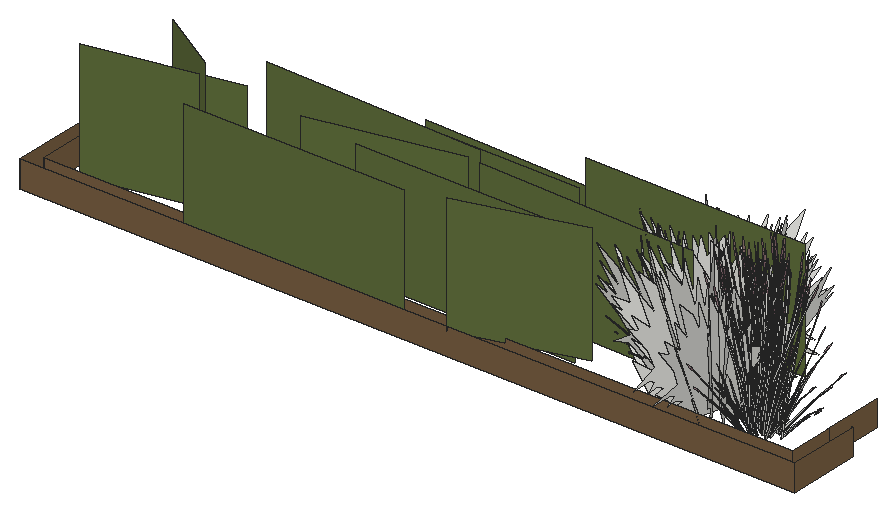
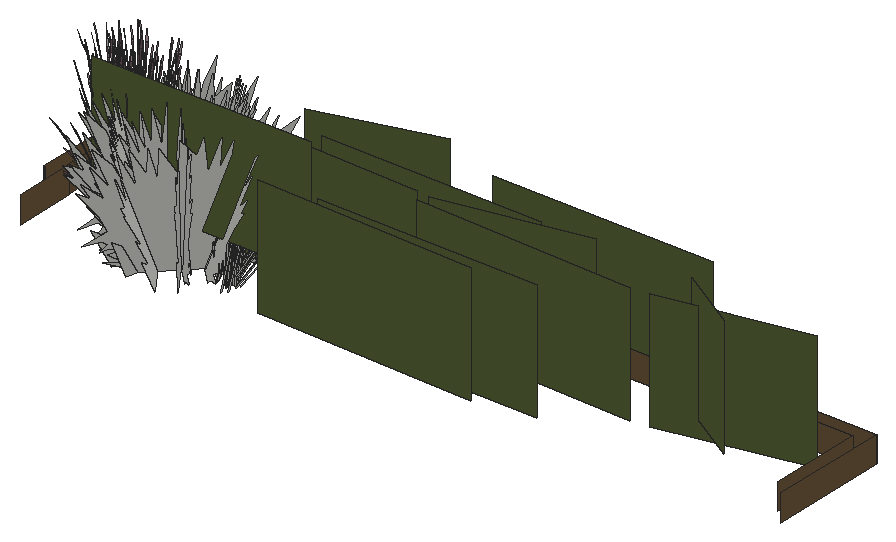
# SketchUp Ruby script. Lengths in inches.
U = 1.inch
M = Sketchup.active_model
def pt(a) = Geom::Point3d.new(a.map { |v| v * U })
def face(e, loops, mat)
  f = e.add_face(loops[0].map { |a| pt(a) })
  loops[1..].each { |l| e.add_face(l.map { |a| pt(a) }).erase! }
  f.material = f.back_material = mat if mat
  f
end
# faces: each face lists its corners as indices into pts; further lists are holes
def faces(e, pts, list, mat = nil) = list.each { |f| face(e, (f[0].is_a?(Array) ? f : [f]).map { |l| l.map { |i| pts[i] } }, mat) }
# xy, xz, yz: faces in a plane at the given z, y or x. An outline is a flat list of corners, or four numbers for a rectangle; further outlines are holes
def ring(l) = l.size == 4 ? [[l[0], l[1]], [l[2], l[1]], [l[2], l[3]], [l[0], l[3]]] : l.each_slice(2).to_a
def flat(e, list, mat, &to3) = list.each { |f| face(e, (f[0].is_a?(Array) ? f : [f]).map { |l| ring(l).map { |u, v| to3.(u, v) } }, mat) }
def xy(e, z, list, mat = nil) = flat(e, list, mat) { |x, y| [x, y, z] }
def xz(e, y, list, mat = nil) = flat(e, list, mat) { |x, z| [x, y, z] }
def yz(e, x, list, mat = nil) = flat(e, list, mat) { |y, z| [x, y, z] }
def lines(e, pts, list) = list.each { |a, b| e.add_line(pt(pts[a]), pt(pts[b])) }
# prism: a flat outline (further loops are holes) pulled along v
def prism(e, loops, v, mat = nil)
  f = face(e, loops, mat); d = Geom::Vector3d.new(v.map { |x| x * U })
  f.pushpull(f.normal.samedirection?(d) ? d.length : -d.length)
end
def box(e, o, s, mat = nil) = prism(e, [[o, [o[0] + s[0], o[1], o[2]], [o[0] + s[0], o[1] + s[1], o[2]], [o[0], o[1] + s[1], o[2]]]], [0, 0, s[2]], mat)
def at(x, y, z, deg = 0) = Geom::Transformation.translation(pt([x, y, z])) * Geom::Transformation.rotation(ORIGIN, Z_AXIS, deg.degrees)
def axes(o, x, y, z) = Geom::Transformation.new([*x, 0, *y, 0, *z, 0, *pt(o).to_a, 1])
def part(name) = M.definitions.add(name)
# library, detail: a bought-in or finely detailed component or shape, given as its bounding box
def library(name, o, s) = part(name).tap { |d| box(d.entities, o, s) }
def detail(e, o, s) = box(e.add_group.entities, o, s)
def put(e, d, t, mat = nil) = e.add_instance(d, t).tap { |i| i.material = mat if mat }
def group(e, t, mat = nil) = e.add_group.tap { |g| g.transformation = t; g.material = mat if mat }.entities
root = M.entities
M.materials.add("Grass2").color = [97, 112, 61]
M.materials.add("LightPink_Translucent").color = [144, 107, 117]
M.materials["LightPink_Translucent"].alpha = 0.75
M.materials.add("Soil_03_1K").color = [122, 96, 67]
c1 = part("blade")
p = [[2.15,0.21,22],[0,0.17,0],[0.09,0.45,0],[2.18,0.31,22],[2.29,0.31,22],[0.38,0.45,0],
  [2.48,0.24,33],[2.49,0.24,33],[2.48,0.22,33]]
faces(c1.entities,p,[[0,1,2,3],[4,5,2,3],[6,3,4,7],[8,0,3,6]])
c2 = part("seeds")
p = [[0.3,-0.1,1.38],[-0.01,-0.03,1.59],[-0.01,-0.03,0.03],[0.14,-0.07,-0.07],[0.29,-0.03,3],[0.15,0.01,3.11]]
faces(c2.entities,p,[[0,1,2,3],[1,0,4,5]],"LightPink_Translucent")
c3 = part("blade with seeds")
put(c3.entities,c1,at(0,0,0))
put(c3.entities,c2,axes([2.4,0.25,30.99],[1.5799,-0.05474,1.17369],[-0.12525,1.92788,0.29478],[-0.07173,-0.02425,1.56792]))
c4 = part("Group\#22")
xz(c4.entities,0,[[0,0,62.37,62.37]],"Grass2")
c5 = part("Grass")
put(c5.entities,c4,at(102.75,113.61,7.86,-130.817))
put(c5.entities,c4,at(63.84,171.21,0.17))
put(c5.entities,c4,at(131.2,149.2,20.75))
put(c5.entities,c4,at(113.26,0,11.94,57.296))
put(c5.entities,c4,at(36.98,10.45,5.02))
put(c5.entities,c4,at(77.99,64.03,5.18))
put(c5.entities,c4,at(168.32,102.22,8.04,171.887))
put(c5.entities,c4,at(142.1,179.07,0,171.887))
put(c5.entities,c4,at(103.38,132.8,9.02,171.887))
put(c5.entities,c4,at(40.77,108.39,1.9,-130.817))
put(c5.entities,c4,at(14.86,142.73,10.93,-73.521))
c6 = part("blade with seeds\#1")
put(c6.entities,c1,at(0,0,0))
c7 = part("Component\#6")
xz(c7.entities,0,[[-7.84,0,-9.38,1.27,-13.33,2.74,-9.72,2.74,-12.46,4.76,-10.42,5.61,-11.09,5.91,-12.29,6.43,-14.04,5.51,-12.66,7.47,-13.79,8.27,-17.41,7.2,-12.68,10.6,-14.36,14.66,-18.8125,20.79,-16.1,19.31,-17.89,23.09,-13.72,19.25,-16.46,27.33,-12.55,21.85,-16.26,31.69,-12.42,27.71,-10.09,22.64,-11.66,30.3,-7.6,21.37,-9.33,31.16,-5.98,24.77,-5.98,31.16,-3.85,22.89,-3.85,31.16,-0.14,24.32,-0.14,32.95,3.15,28.93,4.22,33.24,5.28,24.41,7.5,33.04,7.5,25.47,9.76,32.21,9.01,24.9375,12.04,31.72,9.8,23.08,13.59,31.68,12.3,26.01,15.16,30.22,11.37,20.82,13.73,24.07,13.73,18.79,18.81,26.9375,17.03,20.08,20.56,21.75,18.25,18.3,20.56,20.08,12.54,9.27,16.8,12.66,11.125,4.45,16.74,8.03,13.47,0]])
c8 = part("Component\#7")
xz(c8.entities,0,[[-7.84,0,-9.38,1.27,-13.33,2.74,-9.72,2.74,-12.46,4.76,-10.42,5.61,-11.09,5.91,-12.29,6.43,-14.04,5.51,-12.66,7.47,-13.79,8.27,-17.41,7.2,-12.68,10.6,-14.36,14.66,-18.8125,20.79,-16.1,19.31,-17.89,23.09,-13.72,19.25,-16.46,27.33,-12.55,21.85,-16.26,31.69,-12.42,27.71,-10.09,22.64,-11.66,30.3,-7.6,21.37,-9.33,31.16,-5.98,24.77,-5.98,31.16,-3.85,22.89,-3.85,31.16,-0.14,24.32,-0.14,32.95,3.15,28.93,4.22,33.24,5.28,24.41,7.5,33.04,7.5,25.47,9.76,32.21,9.01,24.9375,12.04,31.72,9.8,23.08,13.59,31.68,12.3,26.01,15.16,30.22,11.37,20.82,13.73,24.07,13.73,18.79,18.81,26.9375,17.03,20.08,20.56,21.75,18.25,18.3,20.56,20.08,12.54,9.27,16.8,12.66,11.125,4.45,16.74,8.03,13.47,0]])
put(c8.entities,c7,axes([0,-4.21,0],[1,0,0],[0,0.96593,0.25882],[0,-0.25882,0.96593]))
c9 = part("Ornamental grass clump")
put(c9.entities,c8,axes([-3.36,-0.02,0],[1.6215,0,0],[0,1.6215,0],[0,0,1.6215]))
put(c9.entities,c8,axes([-0.07,-1.84,0],[-0.93005,1.32826,0],[-1.32826,-0.93005,0],[0,0,1.6215]))
put(c9.entities,c8,axes([1.16,1.19,0],[-1.14657,-1.14657,0],[1.14657,-1.14657,0],[0,0,1.6215]))
put(c9.entities,c8,axes([-0.28,-3,0],[0.41968,1.56625,0],[-1.56625,0.41968,0],[0,0,1.6215]))
put(c9.entities,c8,axes([-2.07,1.56,0],[1.14657,-1.14657,0],[1.14657,1.14657,0],[0,0,1.6215]))
xz(root,49.75,[[307.48,0,600.39,10]],"Soil_03_1K")
xz(root,54.75,[[312.48,0,595.39,10]],"Soil_03_1K")
xz(root,71.87,[[595,0,595.39,10]])
xz(root,76.87,[[600,0,600.39,10]])
yz(root,307.48,[[49.75,0,94.87,10]],"Soil_03_1K")
yz(root,312.48,[[54.75,0,89.87,10]],"Soil_03_1K")
yz(root,595,[[71.87,0,94.87,10]],"Soil_03_1K")
yz(root,595.39,[[54.75,0,71.87,10]],"Soil_03_1K")
yz(root,600.39,[[49.75,0,76.87,10]],"Soil_03_1K")
put(root,c3,axes([572.64,67.23,1.78],[-0.34835,0.20963,1.43002],[-1.04325,-0.36691,-0.30754],[0.19338,-0.4563,0.61141]))
put(root,c3,axes([567.24,66.83,1.78],[-0.07421,0.33879,1.43002],[-1.08488,0.28361,-0.30754],[-0.25359,-0.4379,0.61141]))
put(root,c3,axes([570.04,66.09,0.6875],[-0.20555,0.03731,1.76342],[-1.13672,-0.42002,-0.26939],[0.01907,-0.35034,0.30037]))
put(root,c3,axes([571.35,65.56,1.96],[0.15721,0.60392,1.1486],[-0.87211,-0.33448,0.84392],[0.09385,-0.30923,0.25299]))
put(root,c3,axes([566.87,66.29,1.96],[0.63926,0.36046,1.1486],[-0.93099,0.21668,0.84392],[-0.1992,-0.27702,0.25299]))
put(root,c3,axes([566.36,67.37,0.6875],[-0.11871,0.13643,1.76342],[-1.19964,0.29415,-0.26939],[-0.2898,-0.26759,0.30037]))
put(root,c3,axes([568.34,71.12,1.29],[-0.50328,-1.06202,-0.69835],[1.44974,-0.38248,-0.18329],[-0.05563,-0.35963,1.54149]))
put(root,c3,axes([575.07,67.875,0.6875],[-0.18342,-0.08159,1.76342],[-0.47115,-0.9115,-0.26939],[0.31784,-0.24736,0.30037]))
put(root,c3,axes([568.14,68.07,1.57],[-0.7662,-1.03778,0],[1.28187,-0.57875,-0.51607],[0.29196,-0.13181,1.63711]))
put(root,c3,axes([569.83,66.82,1.32],[-0.84686,0.59414,-0.03893],[-0.77596,-0.65071,-0.17649],[-0.05463,-0.18438,0.58215]))
put(root,c3,axes([565.375,70.97,1.21],[0,-1.03566,-0.49651],[1.37109,0,0],[0,-0.23588,1.57504]))
put(root,c3,axes([569.1875,67.91,1.21],[1.14694,-0.51783,-0.49651],[0.68554,0.92854,0],[0.26122,-0.11794,1.57504]))
put(root,c3,axes([575.99,69.7,1.78],[-0.4378,-0.03068,1.43002],[-0.44851,-0.8229,-0.30754],[0.53783,-0.23279,0.61141]))
put(root,c3,axes([570.55,70.03,1.25],[0.82544,-0.77843,-0.62353],[1.0254,0.70586,-0.16365],[0.33076,-0.19418,1.37633]))
put(root,c3,axes([576.5,68.18,1.96],[-0.40819,0.5272,1.1486],[-0.35086,-0.70831,0.84392],[0.33713,-0.17749,0.25299]))
put(root,c3,axes([569.11,71.4,1.4],[0.59459,-0.93321,-0.44739],[1.23546,0.44912,0.21531],[0,-0.21512,1.43643]))
put(root,c3,axes([569.65,70.93,1.86],[-0.1428,-1.18174,-0.29095],[1.48733,-0.07145,-0.50002],[0.26191,-0.15741,1.59708]))
put(root,c3,axes([565.96,71,1.22],[0.85545,-0.64616,-0.30978],[0.85545,0.64616,0.30978],[0,-0.20813,1.38974]))
put(root,c3,axes([565.62,67.9,1.32],[-0.35352,0.84566,-0.03893],[-1.08806,-0.26014,-0.17649],[-0.1652,-0.13832,0.58215]))
put(root,c3,axes([568.96,72.17,1.86],[-1.38012,-0.49416,-0.29095],[0.66454,-1.04299,-0.50002],[-0.04337,-0.25608,1.59708]))
put(root,c3,axes([565.03,71.76,1.57],[-1.53239,0,0],[0,-1.1575,-0.51607],[0,-0.26363,1.63711]))
put(root,c3,axes([565.29,69.69,1.78],[0.23927,0.28834,1.43002],[-0.55135,0.78376,-0.30754],[-0.56612,-0.18733,0.61141]))
put(root,c3,axes([569.45,68.32,1.22],[1.14332,0.25625,-0.30978],[-0.28787,0.90242,0.30978],[0.23049,-0.10406,1.38974]))
put(root,c3,axes([566.22,71.45,1.52],[-1.1399,0.87071,0.30756],[-1.1406,-0.86155,-0.36492],[-0.03981,-0.24727,1.64885]))
put(root,c3,axes([569.85,71.86,1.625],[1.3808,0.50196,0.24065],[-0.66454,1.04299,0.50002],[0,-0.24043,1.60543]))
put(root,c3,axes([569.31,73.27,1.63],[0.32481,-1.2272,-0.23429],[1.54007,0.21392,0.51271],[-0.26911,-0.16947,1.5644]))
put(root,c3,axes([563.87,70.56,1.96],[0.78239,-0.07411,1.1486],[-0.49629,0.65296,0.84392],[-0.38663,-0.09795,0.25299]))
put(root,c3,axes([569.4,71.16,1.91],[-1.33077,0.06393,0.44739],[-0.12035,-1.06125,-0.21531],[0.23824,-0.10756,1.43643]))
put(root,c3,axes([565.96,71.93,1.67],[0,1.03566,0.49651],[-1.37109,0,0],[0,-0.23588,1.57504]))
put(root,c3,axes([573.79,68.33,1.57],[0.7662,-1.03778,0],[1.28187,0.57875,-0.51607],[0.29196,0.13181,1.63711]))
put(root,c3,axes([569.2,72.77,1.4],[-0.73619,-0.86927,-0.44739],[1.11511,-0.61213,0.21531],[-0.23824,-0.10756,1.43643]))
put(root,c3,axes([569.35,71.54,1.55],[0.53281,1.15808,0.45755],[-1.52239,0.4027,0.17955],[0.01861,-0.2128,1.58856]))
put(root,c3,axes([576.8,72.43,1.17],[-0.7893,0.12429,1.41583],[-0.12563,-0.9893,0.08104],[0.55282,-0.14974,0.80566]))
put(root,c3,axes([578.24,71.55,1.45],[-0.75977,-0.66224,-0.06488],[0.83212,-0.6068,-0.29416],[0.23578,-0.04272,0.97024]))
put(root,c3,axes([569.09,72.45,1.91],[-0.59459,0.93321,0.44739],[-1.23546,-0.44912,-0.21531],[0,-0.21512,1.43643]))
put(root,c3,axes([571.27,71.64,1.4],[0,-1.19833,0],[1.53239,0,0],[0,0,1.79456]))
put(root,c3,axes([573.13,68.87,1.67],[-1.14694,-0.51783,0.49651],[0.68554,-0.92854,0],[0.26122,0.11794,1.57504]))
put(root,c3,axes([568.54,73.1,1.25],[-1.27479,-0.1698,-0.62353],[0.26901,-1.04736,-0.16365],[-0.38043,-0.12691,1.37633]))
put(root,c3,axes([570.54,70.89,1.55],[-1.01611,0.93987,0.45755],[-1.20717,-0.82966,0.17955],[0.24496,-0.0938,1.58856]))
put(root,c3,axes([571.65,72.57,1.49],[-1.1399,-0.8914,-0.06131],[1.1406,-0.89194,0],[-0.03981,-0.03113,1.75571]))
put(root,c3,axes([568.78,69.34,1.67],[-0.35402,1.02926,0.17642],[-1.29548,-0.29127,0.35086],[0.22379,-0.00501,1.60407]))
put(root,c3,axes([568.24,70.17,0.79],[-1.20625,0.41464,1.28929],[-0.38394,-1.1897,0.50096],[0.74071,0.01979,1.46642]))
put(root,c3,axes([571.48,70.48,1.81],[0.23642,-0.92427,0.1448],[1.15506,0.16044,-0.41347],[0.21021,0.09491,1.26744]))
put(root,c3,axes([569.49,72.68,1.55],[1.54892,0.2182,0.45755],[-0.31522,1.23236,0.17955],[-0.22636,-0.119,1.58856]))
put(root,c3,axes([577.66,71.78,0.6875],[-0.06405,-0.15723,1.76342],[0.44421,-0.91974,-0.26939],[0.4481,-0.01323,0.30037]))
put(root,c3,axes([564.44,71.625,0.6875],[0.03108,0.16322,1.76342],[-0.62654,0.85237,-0.26939],[-0.44504,-0.04296,0.30037]))
put(root,c3,axes([570.99,70.73,1.91],[-0.73619,-0.86927,0.44739],[1.11511,-0.61213,-0.21531],[0.23824,0.10756,1.43643]))
put(root,c3,axes([567.1875,74.7,1.22],[-0.28787,-0.90242,-0.30978],[1.14332,-0.25625,0.30978],[-0.23049,-0.10406,1.38974]))
put(root,c3,axes([568.65,74.65,1.67],[1.31687,-0.27488,0.17642],[0.32517,1.02297,0.35086],[-0.11745,-0.14905,1.60407]))
put(root,c3,axes([571.37,70.78,1.86],[1.23732,-0.68758,-0.29095],[0.8228,0.97154,-0.50002],[0.30528,0.09867,1.59708]))
put(root,c3,axes([566.87,75.09,1.21],[-1.14694,-0.51783,-0.49651],[0.68554,-0.92854,0],[-0.26122,-0.11794,1.57504]))
put(root,c3,axes([574.49,68.95,1.21],[1.14694,0.51783,-0.49651],[-0.68554,0.92854,0],[0.26122,0.11794,1.57504]))
put(root,c3,axes([572.31,71.91,1.4],[1.37109,0,0],[0,1.07219,0],[0,0,1.78407]))
put(root,c5,axes([318.24,49.75,0],[1.33,0,0],[0,0.23856,0],[0,0,0.72]))
put(root,c3,axes([569.99,73.26,1.86],[-1.23732,0.68758,-0.29095],[-0.8228,-0.97154,-0.50002],[-0.30528,-0.09867,1.59708]))
put(root,c3,axes([572.7,69.39,1.67],[-1.31687,0.27488,0.17642],[-0.32517,-1.02297,0.35086],[0.11745,0.14905,1.60407]))
put(root,c6,axes([526.6875,81.62,1.03],[-0.2403,0.27843,1.28914],[-0.79492,-0.36227,-0.27724],[0.10768,-0.56334,0.55117]))
put(root,c3,axes([574.17,69.34,1.22],[0.28787,0.90242,-0.30978],[-1.14332,0.25625,0.30978],[0.23049,0.10406,1.38974]))
put(root,c3,axes([571.87,71.36,1.57],[-1.54892,-0.2182,0.49198],[0.31522,-1.23236,0.19306],[0.22636,0.119,1.70813]))
put(root,c3,axes([570.63,74.4,1.4],[-0.39985,-0.89288,0],[1.1418,-0.31268,0],[0,0,1.54371]))
put(root,c3,axes([569.87,73.56,1.81],[-0.23642,0.92427,0.1448],[-1.15506,-0.16044,-0.41347],[-0.21021,-0.09491,1.26744]))
put(root,c3,axes([572.13,74.28,1.38],[1.2866,-0.3514,-0.19198],[0.45209,1.01223,0.00008],[0.14202,-0.03884,1.73897]))
put(root,c3,axes([572.57,74.7,1.67],[0.35402,-1.02926,0.17642],[1.29548,0.29127,0.35086],[-0.22379,0.00501,1.60407]))
put(root,c3,axes([572.28,72.37,1.41],[0.85545,0.66896,0],[-0.85545,0.66896,0],[0,0,1.69266]))
put(root,c3,axes([574.6,72.08,1.67],[-0.96285,-0.75439,0.17642],[0.97031,-0.7317,0.35086],[-0.10634,0.15406,1.60407]))
put(root,c6,axes([525.375,83.18,3.1875],[-0.4315,-1.0159,-0.64046],[0.88824,-0.56616,0.07729],[-0.1009,-0.49086,0.906]))
put(root,c3,axes([572.8125,70.9375,1.25],[1.27479,0.1698,-0.62353],[-0.26901,1.04736,-0.16365],[0.38043,0.12691,1.37633]))
put(root,c3,axes([578.45,72.77,1.96],[-0.75718,0.17097,1.1486],[0.35641,-0.70661,0.84392],[0.40168,0.04835,0.25299]))
put(root,c3,axes([570.35,74.81,1.39],[-1.23546,-0.46496,0],[0.59459,-0.96613,0],[0,0,1.62707]))
put(root,c3,axes([571.375,73.57,1.66],[-1.19666,-0.83357,-0.25192],[1.00694,-0.93603,0.5513],[-0.32224,0.09751,1.68216]))
put(root,c3,axes([568.23,75.17,1.67],[1.14694,0.51783,0.49651],[-0.68554,0.92854,0],[-0.26122,-0.11794,1.57504]))
put(root,c6,axes([524.69,81.02,0.04],[-0.14833,0.06042,1.5897],[-0.86768,-0.41907,-0.24285],[-0.01248,-0.42273,0.27078]))
put(root,c6,axes([525.3,81.83,0.48],[0.11725,0.74462,1.27635],[-0.9333,0.11852,0.07306],[-0.14126,-0.52153,0.72629]))
put(root,c3,axes([572.27,71.59,1.91],[0.59459,-0.93321,0.44739],[1.23546,0.44912,-0.21531],[0,0.21512,1.43643]))
put(root,c3,axes([572.04,72.12,1.48],[0,1.19774,-0.05637],[-1.53239,0,0],[0,0.03764,1.79368]))
put(root,c3,axes([572.15,71.27,1.4],[0.73619,0.86927,-0.44739],[-1.11511,0.61213,0.21531],[0.23824,0.10756,1.43643]))
put(root,c6,axes([527.17,84.17,3.1875],[0.02352,-1.1557,-0.64046],[0.99061,0.07762,0.07729],[0.10454,-0.48961,0.906]))
put(root,c3,axes([567.57,75.71,1.57],[-0.7662,1.03778,0],[-1.28187,-0.57875,-0.51607],[-0.29196,-0.13181,1.63711]))
put(root,c6,axes([525.62,80.28,1.1875],[0.1613,0.71432,1.03545],[-0.66662,-0.33623,0.76078],[0.04561,-0.37895,0.22807]))
put(root,c6,axes([525.46,82.32,2.78],[0.27256,-0.96081,-0.31925],[0.79518,0.28024,0.41216],[-0.07291,-0.38684,0.78863]))
put(root,c6,axes([522.72,82.59,1.03],[-0.02894,0.41302,1.28914],[-0.77632,0.42312,-0.27724],[-0.21961,-0.50739,0.55117]))
put(root,c3,axes([575.39,72.11,1.67],[0,-1.03566,0.49651],[1.37109,0,0],[0,0.23588,1.57504]))
put(root,c3,axes([571.95,72.88,1.91],[1.33077,-0.06393,0.44739],[0.12035,1.06125,-0.21531],[-0.23824,0.10756,1.43643]))
put(root,c3,axes([572.78,71.8,1.81],[1.1418,-0.30203,0.1448],[0.39985,0.86246,-0.41347],[0,0.18981,1.26744]))
put(root,c6,axes([525.05,82.98,2.92],[-0.88873,-0.31321,-0.46065],[0.30463,-1.07385,-0.35681],[-0.08149,-0.43235,0.88141]))
put(root,c3,axes([570.77,73.39,1.4],[-1.33077,0.06393,-0.44739],[-0.12035,-1.06125,0.21531],[-0.23824,0.10756,1.43643]))
put(root,c3,axes([577.03,73.9,1.78],[-0.29514,-0.25472,1.43002],[0.38401,-0.84262,-0.30754],[0.59714,0.11414,0.61141]))
put(root,c3,axes([571.75,74.83,1.4],[1.23546,0.46496,0],[-0.59459,0.96613,0],[0,0,1.74954]))
put(root,c3,axes([572.24,75.85,1.39],[-0.75665,-1.04141,-0.05142],[1.28187,-0.57875,0.51607],[-0.31588,0.09915,1.6363]))
put(root,c3,axes([571.98,73.34,1.81],[0.90538,0.62224,0.1448],[-0.75521,0.70202,-0.41347],[-0.21021,0.09491,1.26744]))
put(root,c6,axes([523.43,83.47,3.1875],[-0.77091,-0.6039,-0.64046],[0.54787,-1.05824,0.07729],[-0.27931,-0.36058,0.906]))
put(root,c6,axes([523.16,82.67,2.78],[-0.13963,-1.00636,-0.31925],[0.79822,-0.26574,0.41216],[-0.2144,-0.28839,0.78863]))
put(root,c6,axes([527.58,83.48,2.78],[0.61172,-0.65782,-0.31925],[0.57907,0.75112,0.41216],[0.08811,-0.38163,0.78863]))
put(root,c3,axes([572.9375,75.25,1.67],[1.14694,-0.51783,0.49651],[0.68554,0.92854,0],[-0.26122,0.11794,1.57504]))
put(root,c3,axes([571.31,74.4375,1.48],[0.53281,1.18979,-0.06012],[-1.52239,0.41691,0],[0.01861,0.04155,1.72173]))
put(root,c3,axes([571.9,75.72,1.22],[-1.14332,-0.25625,-0.30978],[0.28787,-0.90242,0.30978],[-0.23049,0.10406,1.38974]))
put(root,c3,axes([563.65,73.89,1.78],[0.42589,0.08502,1.43002],[0.2745,0.86839,-0.30754],[-0.57851,0.16255,0.61141]))
put(root,c3,axes([576.32,72.28,1.57],[1.53239,0,0],[0,1.1575,-0.51607],[0,0.26363,1.63711]))
put(root,c3,axes([575.71,72.875,1.39],[-1.53164,-0.00828,-0.04976],[0,-1.1575,0.49943],[-0.04813,0.2635,1.58352]))
put(root,c3,axes([572.39,71.87,1.86],[1.38012,0.49416,-0.29095],[-0.66454,1.04299,-0.50002],[0.04337,0.25608,1.59708]))
put(root,c6,axes([524.48,80.47,0.73],[-0.62476,0.71677,-0.05849],[-0.57245,-0.78502,-0.26518],[-0.0403,-0.22243,0.87466]))
put(root,c6,axes([521.3,82.12,1.1875],[0.49736,0.38508,1.03545],[-0.66822,0.331,0.76078],[-0.16744,-0.31805,0.22807]))
put(root,c3,axes([562.76,75.71,1.96],[0.51072,-0.46938,1.1486],[0.20153,0.74307,0.84392],[-0.36908,0.13305,0.25299]))
put(root,c3,axes([575.39,73.04,1.22],[-0.85545,0.64616,-0.30978],[-0.85545,-0.64616,0.30978],[0,0.20813,1.38974]))
put(root,c3,axes([571.7,73.11,1.86],[0.1428,1.18174,-0.29095],[-1.48733,0.07145,-0.50002],[-0.26191,0.15741,1.59708]))
put(root,c3,axes([572.24,72.64,1.4],[-0.59459,0.93321,-0.44739],[-1.23546,-0.44912,0.21531],[0,0.21512,1.43643]))
put(root,c6,axes([523.07,83.5,2.92],[-0.89213,0.297,-0.46065],[-0.15606,-1.12475,-0.35681],[-0.23962,-0.32232,0.88141]))
put(root,c6,axes([523.89,85.59,0.55],[0.16018,-1.20264,-0.5621],[0.98808,0.25378,-0.14753],[0.11973,-0.3589,1.24074]))
put(root,c6,axes([528.97,84.07,0.04],[-0.14106,-0.08423,1.5897],[-0.41543,-1.06044,-0.24285],[0.21501,-0.3215,0.27078]))
put(root,c3,axes([570.81,74.01,1.25],[-0.82544,0.77843,-0.62353],[-1.0254,-0.70586,-0.16365],[-0.33076,0.19418,1.37633]))
put(root,c3,axes([572.28,75.32,1.52],[1.53422,0.33662,0.30756],[-0.38383,1.20322,-0.36492],[-0.25393,0.15059,1.64885]))
put(root,c6,axes([522.02,84.02,0.51],[0.48852,-1.08202,-0.44759],[0.87598,0.64674,0],[0.11126,-0.24644,1.41987]))
put(root,c3,axes([572.17,76.13,1.21],[-1.14694,0.51783,-0.49651],[-0.68554,-0.92854,0],[-0.26122,0.11794,1.57504]))
put(root,c3,axes([575.98,73.07,1.21],[0,1.03566,-0.49651],[-1.37109,0,0],[0,0.23588,1.57504]))
put(root,c6,axes([521.43,84.67,0.84],[-0.97904,-0.72283,0],[0.54599,-1.20931,-0.46523],[0.12435,-0.27543,1.47583]))
put(root,c6,axes([521.01,83.46,0.04],[-0.07697,0.17304,1.5897],[-0.85991,0.44448,-0.24285],[-0.23336,-0.29985,0.27078]))
put(root,c6,axes([528.32,85.72,2.92],[-0.23225,-1.14083,-0.46065],[0.87956,-0.19957,-0.35681],[0.25205,-0.30642,0.88141]))
put(root,c3,axes([574.24,75.22,1.96],[-0.69001,-0.29779,1.1486],[0.89096,-0.30257,0.84392],[0.24031,0.2563,0.25299]))
put(root,c6,axes([523.17,89.9,0.13],[0.39117,1.13797,1.16227],[-1.12236,0.3622,0.45161],[0.01867,-0.69878,1.32195]))
put(root,c3,axes([573.21,75.97,1.57],[0.7662,1.03778,0],[-1.28187,0.57875,-0.51607],[-0.29196,0.13181,1.63711]))
put(root,c6,axes([529.21,84.15,1.1],[-0.03064,0.74138,0.9471],[-0.6508,-0.48961,0.52291],[0.23122,-0.29288,0.74292]))
put(root,c3,axes([574.43,76.32,0.6875],[0.08928,-0.14952,1.76342],[1.12407,-0.44035,-0.26939],[0.34078,0.22791,0.30037]))
put(root,c3,axes([572.55,71.86,2.03],[-0.03348,-0.97511,1.41272],[1.51511,0.25277,0.59816],[-0.35835,0.53357,1.3335]))
put(root,c3,axes([572.94,72.93,1.29],[0.44936,0.94823,-0.69212],[-1.29441,0.3415,-0.18165],[0.04967,0.32109,1.52773]))
put(root,c3,axes([564.11,76.19,0.6875],[0.16438,0.10347,1.76342],[0.27873,0.95868,-0.26939],[-0.36432,0.20444,0.30037]))
put(root,c6,axes([525.16,82.29,0.84],[0,-1.44565,0],[1.09198,0,-0.46523],[0.24871,0,1.47583]))
put(root,c6,axes([523.75,86.96,1.1],[-0.64866,-1.16728,-0.26229],[0.91655,-0.77622,-0.45076],[0.09308,-0.288,1.43974]))
put(root,c6,axes([522.39,84.32,0.52],[0.85134,-0.27158,-0.27926],[0.24175,1.0786,0.27926],[0.09817,-0.21744,1.25283]))
put(root,c3,axes([574.35,76.57,1.86],[-0.78586,-0.03248,1.0506],[0.51898,-0.68985,0.58006],[0.31045,0.24509,0.8241]))
put(root,c6,axes([527.93,84.25,1.1875],[-0.28093,0.65095,1.03545],[-0.28545,-0.84053,0.76078],[0.2418,-0.22671,0.22807]))
put(root,c6,axes([527.63,86.57,1.03],[-0.32388,-0.0204,1.28914],[-0.36177,-0.97496,-0.27724],[0.38765,-0.30097,0.55117]))
put(root,c6,axes([523.04,87.73,0.55],[-0.73437,-0.77871,-0.5621],[0.66591,-0.96736,-0.14753],[-0.18319,-0.31204,1.24074]))
put(root,c6,axes([521.32,84.44,2.78],[-0.51441,-0.78225,-0.31925],[0.58738,-0.7405,0.41216],[-0.29843,-0.11267,0.78863]))
put(root,c9,at(545.84,81.64,0))
put(root,c3,axes([571.78,74.9,1.78],[0.02163,-0.34331,1.43002],[1.03345,-0.38348,-0.30754],[0.31903,0.4109,0.61141]))
put(root,c6,axes([524.21,86.22,0.6875],[0.82007,-0.69452,-0.40331],[0.57748,1.05199,0.1941],[0.10147,-0.22475,1.29492]))
put(root,c3,axes([567.09,77.76,1.96],[-0.03171,-0.6158,1.1486],[0.7925,0.43922,0.84392],[-0.15586,0.29352,0.25299]))
put(root,c6,axes([521.86,84.96,3.1875],[-0.90375,-0.03008,-0.64046],[0.0607,-1.26677,0.07729],[-0.38287,-0.13368,0.906]))
put(root,c6,axes([521.94,85.3,0.93],[-0.48852,1.08202,0.44759],[-0.87598,-0.64674,0],[0.11126,-0.24644,1.41987]))
put(root,c6,axes([527.05,86.24,0.67],[-0.33151,-1.21377,-0.17307],[0.95493,-0.4265,0.00007],[-0.03664,-0.13398,1.56765]))
put(root,c3,axes([569.18,76.29,0.6875],[0.19833,-0.05635,1.76342],[1.19302,0.31018,-0.26939],[0.03489,0.3496,0.30037]))
put(root,c6,axes([525,83.16,0.93],[-0.97703,0,0.44759],[0,-1.29348,0],[0.22253,0,1.41987]))
put(root,c6,axes([523.46,86.85,1.05],[-0.87196,-0.22303,0.13053],[0.15136,-1.08968,-0.37274],[0.08953,-0.19831,1.14258]))
put(root,c6,axes([525.9,82.61,0.51],[0.97703,0,-0.44759],[0,1.29348,0],[0.22253,0,1.41987]))
put(root,c3,axes([566.4375,76.43,2.02],[1.11329,-0.1834,0.06507],[0.25594,0.73887,-0.86304],[-0.07058,0.37403,0.7736]))
put(root,c6,axes([521.04,89.02,0.51],[-0.48852,-1.08202,-0.44759],[0.87598,-0.64674,0],[-0.11126,-0.24644,1.41987]))
put(root,c6,axes([520.4,85.76,1.03],[0.19776,0.32863,1.28914],[-0.34614,0.98419,-0.27724],[-0.43048,-0.18244,0.55117]))
